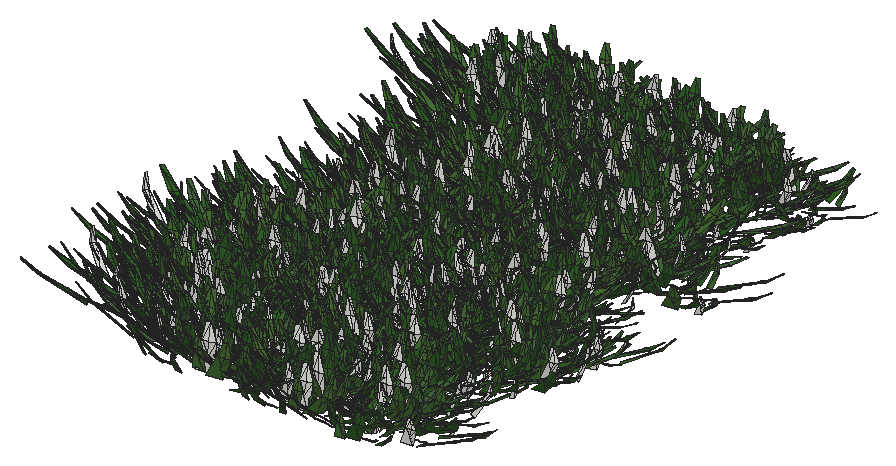
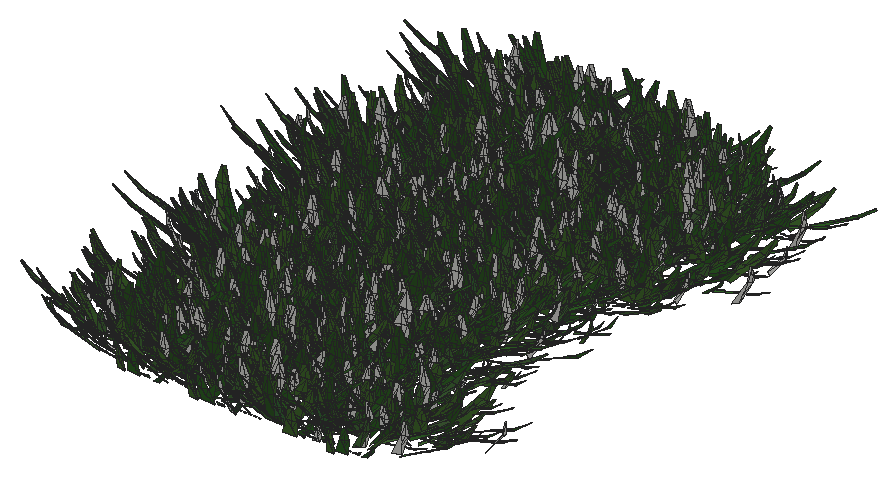
# SketchUp Ruby script. Lengths in inches.
U = 1.inch
M = Sketchup.active_model
def pt(a) = Geom::Point3d.new(a.map { |v| v * U })
def face(e, loops, mat)
  f = e.add_face(loops[0].map { |a| pt(a) })
  loops[1..].each { |l| e.add_face(l.map { |a| pt(a) }).erase! }
  f.material = f.back_material = mat if mat
  f
end
# faces: each face lists its corners as indices into pts; further lists are holes
def faces(e, pts, list, mat = nil) = list.each { |f| face(e, (f[0].is_a?(Array) ? f : [f]).map { |l| l.map { |i| pts[i] } }, mat) }
# xy, xz, yz: faces in a plane at the given z, y or x. An outline is a flat list of corners, or four numbers for a rectangle; further outlines are holes
def ring(l) = l.size == 4 ? [[l[0], l[1]], [l[2], l[1]], [l[2], l[3]], [l[0], l[3]]] : l.each_slice(2).to_a
def flat(e, list, mat, &to3) = list.each { |f| face(e, (f[0].is_a?(Array) ? f : [f]).map { |l| ring(l).map { |u, v| to3.(u, v) } }, mat) }
def xy(e, z, list, mat = nil) = flat(e, list, mat) { |x, y| [x, y, z] }
def xz(e, y, list, mat = nil) = flat(e, list, mat) { |x, z| [x, y, z] }
def yz(e, x, list, mat = nil) = flat(e, list, mat) { |y, z| [x, y, z] }
def lines(e, pts, list) = list.each { |a, b| e.add_line(pt(pts[a]), pt(pts[b])) }
# prism: a flat outline (further loops are holes) pulled along v
def prism(e, loops, v, mat = nil)
  f = face(e, loops, mat); d = Geom::Vector3d.new(v.map { |x| x * U })
  f.pushpull(f.normal.samedirection?(d) ? d.length : -d.length)
end
def box(e, o, s, mat = nil) = prism(e, [[o, [o[0] + s[0], o[1], o[2]], [o[0] + s[0], o[1] + s[1], o[2]], [o[0], o[1] + s[1], o[2]]]], [0, 0, s[2]], mat)
def at(x, y, z, deg = 0) = Geom::Transformation.translation(pt([x, y, z])) * Geom::Transformation.rotation(ORIGIN, Z_AXIS, deg.degrees)
def axes(o, x, y, z) = Geom::Transformation.new([*x, 0, *y, 0, *z, 0, *pt(o).to_a, 1])
def part(name) = M.definitions.add(name)
# library, detail: a bought-in or finely detailed component or shape, given as its bounding box
def library(name, o, s) = part(name).tap { |d| box(d.entities, o, s) }
def detail(e, o, s) = box(e.add_group.entities, o, s)
def put(e, d, t, mat = nil) = e.add_instance(d, t).tap { |i| i.material = mat if mat }
def group(e, t, mat = nil) = e.add_group.tap { |g| g.transformation = t; g.material = mat if mat }.entities
root = M.entities
M.materials.add("Material82").color = [68, 110, 58]
M.materials.add("Material83").color = [48, 90, 38]
M.materials.add("Material84").color = [68, 110, 48]
M.materials.add("Material85").color = [48, 90, 48]
M.materials.add("Material86").color = [58, 110, 58]
M.materials.add("Material87").color = [58, 90, 38]
M.materials.add("Material88").color = [68, 100, 58]
M.materials.add("Material89").color = [48, 100, 38]
c1 = part("grass00")
p = [[-0.6875,0.15,0],[-0.56,0.08,5.52],[-0.04,0.03,2.76],[0.48,-0.02,0],[0.35,-0.02,5.52],[-0.1,-0.14,5.52],
  [-0.12,0.65,8.37],[-0.42,0.65,8.37]]
faces(c1.entities,p,[[0,1,2,3],[3,2,4],[1,5,2],[5,4,2],[1,6,5],[4,5,6],[7,6,1]])
c2 = part("Group16\#1")
put(c2.entities,c1,axes([1.44,-0.61,-0.01],[0.05352,0.12609,0],[-0.10704,0.04543,0.07239],[0.06664,-0.02828,0.11628]),"Material85")
put(c2.entities,c1,axes([0.76,-0.15,-0.01],[0.04676,0.24062,0],[-0.23162,0.04501,0.06642],[0.0652,-0.01267,0.23595]),"Material82")
put(c2.entities,c1,axes([0.79,0.01,-0.01],[-0.00606,0.34651,0],[-0.34381,-0.00602,0.0432],[0.04319,0.00076,0.34386]))
put(c2.entities,c1,axes([1,0.23,-0.01],[-0.07192,0.31144,0],[-0.28722,-0.06632,0.1236],[0.12043,0.02781,0.29478]),"Material84")
put(c2.entities,c1,axes([1.66,0.77,-0.01],[-0.13828,0.29651,0],[-0.21551,-0.1005,0.22471],[0.20365,0.09498,0.23779]),"Material89")
put(c2.entities,c1,axes([0.6875,0.52,-0.01],[-0.18126,0.24051,0],[-0.22746,-0.17142,0.09788],[0.07817,0.05891,0.28481]),"Material84")
put(c2.entities,c1,axes([0.68,0.78,-0.01],[-0.215,0.18688,0],[-0.12385,-0.14248,0.21334],[0.13995,0.16101,0.18878]),"Material82")
put(c2.entities,c1,axes([0.56,1,-0.01],[-0.13756,0.07624,0],[-0.06159,-0.11112,0.0927],[0.04494,0.08108,0.12705]),"Material84")
put(c2.entities,c1,axes([0.2,0.64,-0.01],[-0.23729,0.07254,0],[-0.05711,-0.18681,0.153],[0.04473,0.14632,0.19535]),"Material89")
put(c2.entities,c1,axes([0.0625,0.72,-0.01],[-0.28874,0.02525,0],[-0.02179,-0.24916,0.14647],[0.01276,0.14591,0.25012]),"Material82")
put(c2.entities,c1,axes([-0.08,0.62,-0.01],[-0.34089,-0.04187,0],[0.03255,-0.26504,0.216],[-0.02633,0.21439,0.26703]),"Material89")
put(c2.entities,c1,axes([-0.34,0.98,-0.01],[-0.14314,-0.0493,0],[0.04397,-0.12769,0.06843],[-0.02228,0.0647,0.13505]),"Material89")
put(c2.entities,c1,axes([-0.87,1.45,-0.01],[-0.23488,-0.14114,0],[0.13761,-0.22901,0.06087],[-0.03135,0.05217,0.26717]))
put(c2.entities,c1,axes([-0.72,0.77,-0.01],[-0.14208,-0.13251,0],[0.07209,-0.0773,0.16301],[-0.11118,0.11922,0.1057]),"Material89")
put(c2.entities,c1,axes([-0.62,0.43,-0.01],[-0.14845,-0.21203,0],[0.18654,-0.13061,0.12304],[-0.10079,0.07057,0.22772]),"Material82")
put(c2.entities,c1,axes([-0.68,0.29,-0.01],[-0.13639,-0.32136,0],[0.31723,-0.13464,0.05579],[-0.05136,0.0218,0.34462]),"Material83")
put(c2.entities,c1,axes([-0.64,0.125,-0.01],[-0.0458,-0.23569,0],[0.22124,-0.043,0.08276],[-0.08124,0.01579,0.22538]),"Material86")
put(c2.entities,c1,axes([-1.6,-0.03,-0.01],[0.00576,-0.32897,0],[0.27526,0.00482,0.18018],[-0.18015,-0.00315,0.2753]),"Material84")
put(c2.entities,c1,axes([-1.36,-0.31,-0.01],[0.05718,-0.24765,0],[0.18172,0.04196,0.17267],[-0.16825,-0.03885,0.1865]),"Material89")
put(c2.entities,c1,axes([-1.54,-0.72,-0.01],[0.06537,-0.14017,0],[0.13555,0.06321,0.03939],[-0.0357,-0.01665,0.14956]))
put(c2.entities,c1,axes([-1.19,-0.9,-0.01],[0.09597,-0.12735,0],[0.11214,0.08451,0.07557],[-0.06035,-0.04548,0.14042]),"Material88")
put(c2.entities,c1,axes([-0.47,-0.54,-0.01],[0.11588,-0.10072,0],[0.0618,0.0711,0.12124],[-0.07953,-0.0915,0.0942]))
put(c2.entities,c1,axes([-0.47,-0.84,-0.01],[0.11927,-0.0661,0],[0.06603,0.11913,0.00646],[-0.00313,-0.00565,0.13621]),"Material84")
put(c2.entities,c1,axes([-0.38,-1.24,-0.01],[0.28037,-0.08571,0],[0.0618,0.20215,0.20315],[-0.05939,-0.19428,0.21139]),"Material88")
put(c2.entities,c1,axes([-0.06,-0.66,-0.01],[0.22719,-0.01987,0],[0.01247,0.14255,0.17758],[-0.01547,-0.17691,0.1431]),"Material87")
put(c2.entities,c1,axes([0.11,-0.89,-0.01],[0.14882,0.01828,0],[-0.01058,0.08611,0.12229],[0.01491,-0.12138,0.08676]),"Material85")
put(c2.entities,c1,axes([0.25,-0.72,-0.01],[0.20481,0.07053,0],[-0.06206,0.18022,0.10291],[0.03351,-0.0973,0.1906]),"Material85")
put(c2.entities,c1,axes([0.85,-1.42,-0.01],[0.16481,0.09904,0],[-0.09472,0.15762,0.05616],[0.02893,-0.04814,0.18389]),"Material84")
put(c2.entities,c1,axes([1.01,-1.09,-0.01],[0.21858,0.20385,0],[-0.17495,0.1876,0.15339],[0.10462,-0.11218,0.25652]),"Material89")
put(c2.entities,c1,axes([1.01,-0.71,-0.01],[0.08733,0.12473,0],[-0.06445,0.04512,0.13037],[0.1068,-0.07477,0.07867]),"Material85")
c3 = part("Group15\#1")
put(c3.entities,c2,at(0,0,0))
c4 = part("3darcstudiotree_grass00\#1")
put(c4.entities,c3,at(0,0,0))
put(root,c4,axes([684.42,956.72,-29.74],[2.78328,1.41625,0],[-3.60575,1.10211,-0.03267],[-0.14651,0.04478,1.93988]))
put(root,c4,axes([684.58,991.06,-29.74],[1.42302,1.52353,0],[-4.19442,0.60932,-0.04046],[-0.17686,0.02569,1.56076]))
put(root,c4,axes([684.6875,952.4375,-29.74],[0.02685,1.39613,0],[-4.67009,0.01397,-0.03677],[-0.14547,0.00044,1.38481]))
put(root,c4,axes([686.42,944.23,-29.74],[-3.90096,-0.14279,0],[0.42836,-1.82008,-0.06502],[0.0247,-0.10495,1.42798]))
put(root,c4,axes([685.47,961.63,-29.74],[-0.58657,1.2788,0],[-3.43074,-0.24475,-0.01415],[-0.07642,-0.00545,1.43376]))
put(root,c4,axes([686.5,950.95,-29.74],[1.37504,-1.64012,0],[4.21946,0.55019,-0.04027],[0.19656,0.02563,1.71232]))
put(root,c4,axes([686.58,992.02,-29.74],[3.4755,-0.56156,0],[1.30477,1.25594,-0.00746],[0.01674,0.01612,1.52751]))
put(root,c4,axes([686.01,945.99,-29.74],[2.831,1.13552,0],[-3.26481,1.26594,-0.00938],[-0.03813,0.01479,1.95578]))
put(root,c4,axes([688.69,963.81,-29.74],[-0.94888,-1.39552,0],[4.53946,-0.48005,-0.04199],[0.20499,-0.02168,1.7807]))
put(root,c4,axes([689.05,970.1875,-29.74],[-2.56412,-1.04956,0],[2.92241,-1.11041,-0.03217],[0.12075,-0.04588,1.58546]))
put(root,c4,axes([688.75,950.78,-29.74],[-4.23608,0.30685,0],[-0.85226,-1.82987,-0.05609],[-0.05564,-0.11947,1.94158]))
put(root,c4,axes([689,960.52,-29.74],[-3.83901,-0.76558,0],[1.48905,-1.16132,-0.0255],[0.09039,-0.0705,1.94297]))
put(root,c4,axes([688.6875,996.64,-29.74],[-3.22115,0.33319,0],[-1.15137,-1.73117,-0.03948],[-0.04657,-0.07003,1.58152]))
put(root,c4,axes([688.66,988.74,-29.74],[-3.56945,0.98002,0],[-2.54129,-1.43957,-0.02528],[-0.0766,-0.04339,1.76765]))
put(root,c4,axes([688.42,947.1,-29.74],[0.13943,1.51336,0],[-3.52829,0.05056,-0.04285],[-0.2957,0.00424,1.82733]))
put(root,c4,axes([688.6,986.46,-29.74],[3.38923,-0.39007,0],[1.26949,1.71555,-0.04654],[0.05157,0.06969,1.34343]))
put(root,c4,axes([688.34,994.52,-29.74],[3.63174,0.64343,0],[-1.49454,1.312,-0.04301],[-0.1083,0.09507,1.6797]))
put(root,c4,axes([688.91,961.37,-29.74],[3.52935,-0.50726,0],[1.49485,1.61761,-0.06136],[0.11602,0.12555,1.80687]))
put(root,c4,axes([690.3,948.92,-29.74],[-0.52019,-1.47295,0],[3.61124,-0.19836,-0.01078],[0.07028,-0.00386,1.79898]))
put(root,c4,axes([690.66,972.49,-29.74],[-1.338,-1.30891,0],[3.60545,-0.57321,-0.00075],[0.00363,-0.00058,1.52674]))
put(root,c4,axes([689.23,953.74,-29.74],[3.75686,0.07381,0],[-0.21994,1.74119,-0.00527],[-0.00126,0.00998,1.59512]))
put(root,c4,axes([691.34,992.26,-29.74],[-1.97999,-1.67359,0],[3.87039,-0.71217,-0.01753],[0.07436,-0.01368,1.49864]))
put(root,c4,axes([690.15,980.1,-29.74],[3.4977,-1.17788,0],[2.34178,1.08154,-0.01134],[0.04108,0.01897,1.5074]))
put(root,c4,axes([690.89,945.17,-29.74],[-4.29885,0.51765,0],[-1.3445,-1.73657,-0.03433],[-0.03931,-0.05078,1.35329]))
put(root,c4,axes([690.68,974.28,-29.74],[-3.01219,1.1686,0],[-2.47695,-0.99299,-0.0233],[-0.1132,-0.04538,1.83382]))
put(root,c4,axes([690.42,977.27,-29.74],[-0.71352,1.56405,0],[-4.14814,-0.29432,-0.02584],[-0.10481,-0.00744,1.30174]))
put(root,c4,axes([691.58,983.25,-29.74],[1.98892,-1.13086,0],[3.89758,1.06614,-0.02169],[0.07891,0.02158,1.57389]))
put(root,c4,axes([690.73,955.29,-29.74],[-0.64515,1.28427,0],[-4.09885,-0.32024,-0.03573],[-0.18751,-0.01465,1.67549]))
put(root,c4,axes([692.125,941.89,-29.74],[-3.41936,-0.32293,0],[0.80872,-1.33182,-0.00326],[0.00565,-0.00931,1.93944]))
put(root,c4,axes([690.63,957.94,-29.74],[2.80686,0.98493,0],[-2.35719,1.04478,-0.00943],[-0.03285,0.01456,1.39243]))
put(root,c4,axes([691.37,965.74,-29.74],[-0.90085,1.67926,0],[-4.44806,-0.37112,-0.05558],[-0.25392,-0.02119,1.59125]))
put(root,c4,axes([692.08,989.9,-29.74],[1.68218,-1.47179,0],[3.03421,0.53937,-0.02223],[0.13236,0.02353,1.62899]))
put(root,c4,axes([692.16,980.9,-29.74],[3.50844,-0.55754,0],[1.25662,1.22985,-0.02314],[0.04614,0.04516,1.34449]))
put(root,c4,axes([691.64,968.23,-29.74],[1.7612,1.59038,0],[-3.40002,0.5856,-0.01938],[-0.1015,0.01748,1.58937]))
put(root,c4,axes([693.83,960.2,-29.74],[-1.60359,-1.29455,0],[3.30864,-0.63743,-0.0349],[0.20941,-0.04034,1.84302]))
put(root,c4,axes([694.41,973.52,-29.74],[-3.86108,-0.00922,0],[0.0279,-1.817,-0.0591],[0.00158,-0.1028,1.52309]))
put(root,c4,axes([694.61,969.26,-29.74],[-4.30049,-0.14117,0],[0.33609,-1.59238,-0.036],[0.01919,-0.09092,1.9513]))
put(root,c4,axes([694.39,985.21,-29.74],[1.67099,-1.73753,0],[3.10475,0.46439,-0.00605],[0.0444,0.00664,1.95327]))
put(root,c4,axes([694.48,997.1,-29.74],[1.32812,-1.21732,0],[3.65511,0.62022,-0.02985],[0.14197,0.02409,1.54439]))
put(root,c4,axes([694.19,980.74,-29.74],[0.83797,-1.39271,0],[3.20742,0.30015,-0.04624],[0.35526,0.03324,1.95114]))
put(root,c4,axes([694.18,990.49,-29.74],[-2.03219,1.40442,0],[-2.95743,-0.66557,-0.04437],[-0.22116,-0.04977,1.46464]))
put(root,c4,axes([693.83,948.75,-29.74],[-0.97814,1.51943,0],[-3.80237,-0.3807,-0.01715],[-0.08253,-0.00826,1.46021]))
put(root,c4,axes([695.4,974.73,-29.74],[-0.67683,-1.69031,0],[4.16932,-0.25965,-0.01303],[0.08012,-0.00499,1.96953]))
put(root,c4,axes([695.08,940.56,-29.74],[1.22394,-1.54587,0],[4.34445,0.53497,-0.04262],[0.21661,0.02667,1.81655]))
put(root,c4,axes([695.68,963.42,-29.74],[-4.29208,0.36507,0],[-0.8528,-1.5594,-0.00845],[-0.00798,-0.0146,1.35873]))
put(root,c4,axes([695.14,953.15,-29.74],[-2.45653,1.59128,0],[-3.13753,-0.75331,-0.03488],[-0.14833,-0.03561,1.37068]))
put(root,c4,axes([694.69,958.01,-29.74],[3.38301,-0.17676,0],[0.47183,1.40447,-0.04905],[0.03546,0.10554,1.48186]))
put(root,c4,axes([695.35,966.33,-29.74],[-2.91157,1.30067,0],[-2.86972,-0.9991,-0.01581],[-0.05499,-0.01914,1.33135]))
put(root,c4,axes([695.3125,945.11,-29.74],[3.20776,-0.47754,0],[1.28857,1.34619,-0.04981],[0.10847,0.11332,1.68613]))
put(root,c4,axes([696.54,945.81,-29.74],[-0.83396,-1.47678,0],[3.24144,-0.28469,-0.00779],[0.04244,-0.00373,1.38852]))
put(root,c4,axes([696.57,971.18,-29.74],[-2.06199,-1.44492,0],[3.43124,-0.76156,-0.05229],[0.2544,-0.05646,1.64764]))
put(root,c4,axes([696.67,955.42,-29.74],[0.41064,-1.32496,0],[4.30887,0.2077,-0.02785],[0.12721,0.00613,1.49696]))
put(root,c4,axes([695.76,962.01,-29.74],[-2.19345,1.65823,0],[-4.03021,-0.82913,-0.04188],[-0.20563,-0.0423,1.88687]))
put(root,c4,axes([695.14,983.93,-29.74],[2.88531,0.9286,0],[-2.55752,1.23593,-0.03119],[-0.12387,0.05986,1.90467]))
put(root,c4,axes([696.28,994.86,-29.74],[-1.83042,1.58988,0],[-3.0568,-0.54735,-0.0444],[-0.26156,-0.04683,1.62807]))
put(root,c4,axes([696.62,976.625,-29.74],[-2.26778,1.36387,0],[-3.7802,-0.97758,-0.05216],[-0.16857,-0.04359,1.30947]))
put(root,c4,axes([696.61,978.76,-29.74],[-1.84352,1.61201,0],[-4.26993,-0.75947,-0.03185],[-0.15055,-0.02678,1.82087]))
put(root,c4,axes([696.71,951.04,-29.74],[2.07706,1.01263,0],[-2.63538,0.84072,-0.02717],[-0.1514,0.0483,1.82093]))
put(root,c4,axes([696.81,942.21,-29.74],[3.46015,0.38109,0],[-0.88814,1.25417,-0.03829],[-0.05842,0.0825,1.40372]))
put(root,c4,axes([697.32,988.56,-29.74],[3.97524,-0.29729,0],[0.87691,1.8237,-0.05959],[0.04913,0.10217,1.56123]))
put(root,c4,axes([697.45,991.9375,-29.74],[0.81482,1.77329,0],[-4.44159,0.31742,-0.02342],[-0.11628,0.00831,1.70718]))
put(root,c4,axes([699.55,941.86,-29.74],[-3.61082,-0.39433,0],[1.20081,-1.71014,-0.02644],[0.03989,-0.05681,1.9068]))
put(root,c4,axes([700.26,981.76,-29.74],[-3.88555,-0.79581,0],[2.02489,-1.53765,-0.03725],[0.08107,-0.06156,1.55507]))
put(root,c4,axes([699.46,994.47,-29.74],[-2.70631,1.45447,0],[-3.636,-1.05223,-0.06171],[-0.25363,-0.0734,1.72322]))
put(root,c4,axes([699.21,987.51,-29.74],[1.70731,1.1244,0],[-2.88773,0.68196,-0.04808],[-0.30467,0.07195,1.86326]))
put(root,c4,axes([699.18,970.15,-29.74],[4.38861,-0.21228,0],[0.43057,1.38444,-0.03723],[0.02239,0.072,1.30959]))
put(root,c4,axes([700.52,990.03,-29.74],[0.3333,-1.68825,0],[3.84573,0.11808,-0.01871],[0.11577,0.00355,1.79426]))
put(root,c4,axes([701.04,973.2,-29.74],[-2.17802,-1.23467,0],[3.55396,-0.97507,-0.03629],[0.13271,-0.03641,1.44541]))
put(root,c4,axes([701.14,968.3,-29.74],[-2.33047,-0.97071,0],[3.43186,-1.28143,-0.06171],[0.20646,-0.07709,1.63202]))
put(root,c4,axes([701.34,946.09,-29.74],[0.8669,-1.63737,0],[4.38165,0.36081,-0.01659],[0.07514,0.00619,1.55232]))
put(root,c4,axes([701.89,984.53,-29.74],[-4.08688,-0.61044,0],[1.62889,-1.6961,-0.00084],[0.00115,-0.0012,1.34285]))
put(root,c4,axes([701.1,979.54,-29.74],[-2.729,0.78907,0],[-2.0311,-1.09252,-0.03589],[-0.15909,-0.08558,1.93035]))
put(root,c4,axes([700.56,977.77,-29.74],[3.45505,-0.2676,0],[0.73895,1.48387,-0.00241],[0.00289,0.0058,1.79003]))
put(root,c4,axes([701.05,975.52,-29.74],[-1.50877,1.48911,0],[-3.61563,-0.56976,-0.0529],[-0.26655,-0.042,1.58349]))
put(root,c4,axes([700.54,956.99,-29.74],[1.39252,1.41751,0],[-3.18673,0.48689,-0.02409],[-0.14094,0.02153,1.60735]))
put(root,c4,axes([700.43,944.65,-29.74],[4.57837,0.42186,0],[-0.79113,1.33536,-0.04207],[-0.04884,0.08244,1.32997]))
put(root,c4,axes([701.67,952.64,-29.74],[-2.78854,1.36928,0],[-2.88748,-0.91457,-0.04358],[-0.20411,-0.06465,1.66757]))
put(root,c4,axes([700.97,966.02,-29.74],[3.59081,0.56064,0],[-1.39714,1.39174,-0.03237],[-0.06842,0.06816,1.63378]))
put(root,c4,axes([702.09,996.53,-29.74],[-3.54904,1.16368,0],[-2.54993,-1.20953,-0.00935],[-0.03236,-0.01535,1.61847]))
put(root,c4,axes([701.9,963.43,-29.74],[3.39127,-1.14999,0],[2.14538,0.98397,-0.0226],[0.09906,0.04544,1.65792]))
put(root,c4,axes([703.03,986.53,-29.74],[-4.21718,-0.04667,0],[0.09647,-1.35575,-0.03959],[0.00846,-0.11883,1.96257]))
put(root,c4,axes([701.5,962,-29.74],[4.10063,0.83805,0],[-2.12312,1.61572,-0.0509],[-0.10915,0.08307,1.61215]))
put(root,c4,axes([702.19,960.24,-29.74],[3.6923,-0.26906,0],[0.83055,1.77269,-0.01263],[0.0116,0.02476,1.73191]))
put(root,c4,axes([702.87,951.2,-29.74],[2.76982,-1.52047,0],[2.85461,0.80878,-0.0087],[0.04308,0.01221,1.60603]))
put(root,c4,axes([703.11,955.36,-29.74],[3.07151,-0.57195,0],[1.60637,1.34169,-0.03456],[0.08725,0.07287,1.66747]))
put(root,c4,axes([703.2,991.79,-29.74],[-0.75802,1.26839,0],[-3.28645,-0.30547,-0.04738],[-0.26314,-0.02446,1.4441]))
put(root,c4,axes([702.51,949.48,-29.74],[2.67266,1.37649,0],[-3.28703,0.99263,-0.02004],[-0.06999,0.02114,1.3651]))
put(root,c4,axes([704.77,996.91,-29.74],[-3.58911,0.17625,0],[-0.41421,-1.31187,-0.03309],[-0.02615,-0.08283,1.60704]))
put(root,c4,axes([705.19,977.36,-29.74],[-3.53984,-0.54558,0],[1.35048,-1.36277,-0.02269],[0.0488,-0.04924,1.64292]))
put(root,c4,axes([704.99,950.69,-29.74],[-4.11453,0.51388,0],[-1.13165,-1.40923,-0.01419],[-0.02668,-0.03323,1.75006]))
put(root,c4,axes([704.8125,940.28,-29.74],[2.17079,-1.3067,0],[3.53732,0.91396,-0.04807],[0.21538,0.05565,1.69791]))
put(root,c4,axes([704.98,964.18,-29.74],[2.51974,-1.17528,0],[3.05999,1.02034,-0.03628],[0.13748,0.04584,1.49031]))
put(root,c4,axes([705.78,985.46,-29.74],[-1.7024,-1.44396,0],[3.0538,-0.55996,-0.04244],[0.29035,-0.05324,1.90455]))
put(root,c4,axes([705.8,942.14,-29.74],[1.63405,-1.64828,0],[3.24927,0.50099,-0.00888],[0.05923,0.00913,1.87213]))
put(root,c4,axes([704.86,943.67,-29.74],[-1.01765,1.47435,0],[-4.56253,-0.4898,-0.0223],[-0.09653,-0.01036,1.58974]))
put(root,c4,axes([706.49,992.84,-29.74],[-0.95803,-1.53129,0],[3.44538,-0.33525,-0.01268],[0.07432,-0.00723,1.60602]))
put(root,c4,axes([706.95,965.75,-29.74],[-1.89774,-1.54823,0],[3.70179,-0.70571,-0.04214],[0.19197,-0.0366,1.55921]))
put(root,c4,axes([706.22,987.47,-29.74],[-2.99752,0.92431,0],[-2.30263,-1.1614,-0.02144],[-0.09164,-0.04622,1.94421]))
put(root,c4,axes([705.64,972.62,-29.74],[-0.63419,1.43243,0],[-3.71512,-0.25582,-0.03794],[-0.18856,-0.01298,1.42617]))
put(root,c4,axes([706.2,948.26,-29.74],[-1.88196,1.3957,0],[-3.10758,-0.65171,-0.04799],[-0.32006,-0.06712,1.99284]))
put(root,c4,axes([707.24,958.05,-29.74],[-1.98727,-1.58329,0],[3.14557,-0.61406,-0.01272],[0.05955,-0.01163,1.37453]))
put(root,c4,axes([707.01,994.26,-29.74],[0.20206,-1.72347,0],[4.27325,0.07792,-0.04434],[0.21389,0.0039,1.54852]))
put(root,c4,axes([707.88,959.95,-29.74],[-2.8282,-0.92386,0],[2.41261,-1.14869,-0.01497],[0.06145,-0.02926,1.82381]))
put(root,c4,axes([706.4375,945.9,-29.74],[-1.66334,1.46333,0],[-4.128,-0.72978,-0.00369],[-0.01567,-0.00277,1.57624]))
put(root,c4,axes([707.17,955.7,-29.74],[-3.33624,1.28886,0],[-2.34327,-0.94338,-0.00183],[-0.00717,-0.00289,1.40539]))
put(root,c4,axes([707,979.55,-29.74],[-2.28466,1.61729,0],[-3.8326,-0.84205,-0.0557],[-0.22938,-0.0504,1.55009]))
put(root,c4,axes([708.27,983.32,-29.74],[-3.20918,-1.37059,0],[3.45166,-1.25697,-0.04946],[0.15315,-0.05577,1.48426]))
put(root,c4,axes([708.08,969.96,-29.74],[-4.01536,-0.24387,0],[0.54359,-1.39202,-0.03709],[0.03558,-0.0911,1.68681]))
put(root,c4,axes([707.74,968.24,-29.74],[-3.12054,0.56833,0],[-1.82234,-1.55622,-0.05064],[-0.09583,-0.08183,1.47033]))
put(root,c4,axes([708.49,953.34,-29.74],[0.84647,-1.73268,0],[3.98325,0.30265,-0.00212],[0.01137,0.00086,1.6588]))
put(root,c4,axes([707.9,990.19,-29.74],[3.17331,-0.50017,0],[1.66687,1.64477,-0.02256],[0.03879,0.03827,1.55958]))
put(root,c4,axes([708.39,980.79,-29.74],[1.96831,-1.06776,0],[3.09361,0.88694,-0.02782],[0.14847,0.04257,1.89124]))
put(root,c4,axes([707.86,962.45,-29.74],[2.38559,0.94842,0],[-2.99836,1.17298,-0.03885],[-0.13848,0.05417,1.58937]))
put(root,c4,axes([708.41,975.67,-29.74],[3.11027,0.45791,0],[-1.48719,1.57105,-0.03179],[-0.06172,0.0652,1.76952]))
put(root,c4,axes([710.32,970.99,-29.74],[-1.60231,-1.37282,0],[3.29691,-0.59848,-0.04546],[0.27162,-0.04931,1.78943]))
put(root,c4,axes([710.67,973.1,-29.74],[0.96155,-1.39333,0],[3.31195,0.35548,-0.01758],[0.11319,0.01215,1.71636]))
put(root,c4,axes([711.05,951.07,-29.74],[-3.63945,-0.58666,0],[1.30533,-1.25945,-0.04864],[0.1019,-0.09832,1.4319]))
put(root,c4,axes([711.17,980.76,-29.74],[-1.71956,-1.37213,0],[4.12265,-0.80354,-0.04891],[0.23955,-0.04669,1.88309]))
put(root,c4,axes([711.41,994.17,-29.74],[-3.8816,-0.56323,0],[1.5517,-1.6632,-0.01333],[0.02356,-0.02525,1.7245]))
put(root,c4,axes([710.73,996.82,-29.74],[-3.46015,1.06405,0],[-2.06953,-1.04669,-0.02241],[-0.08068,-0.04081,1.47722]))
put(root,c4,axes([710.99,948.7,-29.74],[-0.53843,-1.61653,0],[3.48383,-0.18047,-0.04534],[0.27707,-0.01435,1.62314]))
put(root,c4,axes([711.37,961.84,-29.74],[0.02414,-1.32822,0],[3.48081,0.00984,-0.01704],[0.11733,0.00033,1.79616]))
put(root,c4,axes([710.19,991.89,-29.74],[-1.06746,1.42925,0],[-3.87706,-0.45036,-0.01201],[-0.05554,-0.00645,1.46096]))
put(root,c4,axes([711.76,967.68,-29.74],[-1.25473,-1.49042,0],[3.70912,-0.48565,-0.03393],[0.14523,-0.01902,1.3212]))
put(root,c4,axes([710.67,940.29,-29.74],[4.07054,-0.47424,0],[1.26442,1.68794,-0.05518],[0.08285,0.1106,1.77288]))
put(root,c4,axes([712.25,944.52,-29.74],[0.9992,-1.70874,0],[3.78612,0.34433,-0.00305],[0.01806,0.00164,1.76865]))
put(root,c4,axes([711.43,964.62,-29.74],[-2.38248,1.06709,0],[-3.21771,-1.11734,-0.02335],[-0.09118,-0.03166,1.67208]))
put(root,c4,axes([710.75,983.89,-29.74],[0.13535,1.36053,0],[-4.14262,0.0641,-0.00595],[-0.03791,0.00059,1.98232]))
put(root,c4,axes([711.87,985.67,-29.74],[-3.44248,1.19972,0],[-2.84327,-1.26888,-0.04086],[-0.12277,-0.05479,1.46035]))
put(root,c4,axes([712.11,965.7,-29.74],[2.50615,-1.32245,0],[2.94011,0.86656,-0.03861],[0.1979,0.05833,1.76068]))
put(root,c4,axes([712.87,945.85,-29.74],[0.83554,-1.66698,0],[4.46376,0.34798,-0.04547],[0.22573,0.0176,1.72572]))
put(root,c4,axes([712.65,990.65,-29.74],[-3.77371,1.09403,0],[-2.05317,-1.10148,-0.00523],[-0.01755,-0.00942,1.47184]))
put(root,c4,axes([712.68,975.46,-29.74],[-3.53362,0.69285,0],[-1.78137,-1.413,-0.01143],[-0.02296,-0.01821,1.35283]))
put(root,c4,axes([711.8,955.1,-29.74],[3.52761,0.55067,0],[-1.26989,1.26523,-0.04887],[-0.1287,0.12823,1.85053]))
put(root,c4,axes([713.6875,957.66,-29.74],[-4.29343,-0.7683,0],[1.85419,-1.61153,-0.00153],[0.00342,-0.00297,1.82565]))
put(root,c4,axes([713.42,942.29,-29.74],[-4.08016,-0.15242,0],[0.34321,-1.42893,-0.02721],[0.0124,-0.05162,1.31849]))
put(root,c4,axes([712.36,978.6,-29.74],[1.28441,1.48375,0],[-3.48852,0.46968,-0.04031],[-0.24472,0.03295,1.77227]))
put(root,c4,axes([713.39,988.62,-29.74],[-3.58514,0.47051,0],[-1.41535,-1.67729,-0.02244],[-0.03437,-0.04073,1.62972]))
put(root,c4,axes([713.72,960.4375,-29.74],[0.26653,-1.73376,0],[4.03869,0.09656,-0.02606],[0.1443,0.00345,1.68211]))
put(root,c4,axes([713.45,953.66,-29.74],[-2.42435,1.35441,0],[-3.23148,-0.89962,-0.04566],[-0.20763,-0.0578,1.65042]))
put(root,c4,axes([714.21,977.57,-29.74],[3.81611,-0.29546,0],[0.81359,1.63432,-0.02697],[0.02626,0.05275,1.59996]))
put(root,c4,axes([716.48,962.01,-29.74],[-4.03021,-0.53258,0],[1.1352,-1.33605,-0.02118],[0.04192,-0.04934,1.66873]))
put(root,c4,axes([716.95,956.72,-29.74],[0.48715,-1.38403,0],[3.63737,0.19912,-0.0013],[0.00869,0.00048,1.85519]))
put(root,c4,axes([716.32,993.95,-29.74],[-1.21919,1.74404,0],[-3.47137,-0.37742,-0.03305],[-0.15949,-0.01734,1.35106]))
put(root,c4,axes([716.89,975.37,-29.74],[-2.03127,1.47153,0],[-3.87167,-0.83121,-0.05406],[-0.22119,-0.04749,1.53936]))
